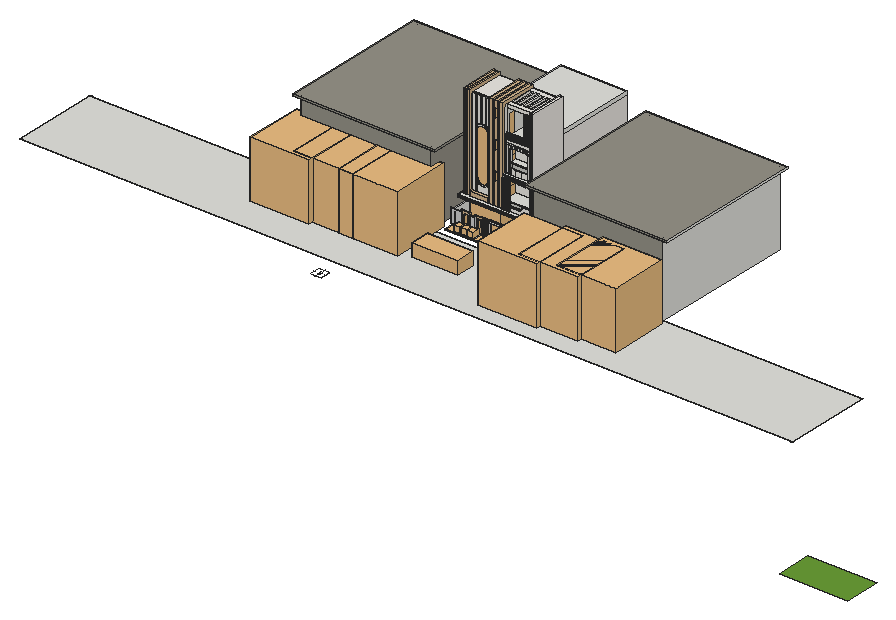
# SketchUp Ruby script. Lengths in inches.
U = 1.inch
M = Sketchup.active_model
def pt(a) = Geom::Point3d.new(a.map { |v| v * U })
def face(e, loops, mat)
  f = e.add_face(loops[0].map { |a| pt(a) })
  loops[1..].each { |l| e.add_face(l.map { |a| pt(a) }).erase! }
  f.material = f.back_material = mat if mat
  f
end
# faces: each face lists its corners as indices into pts; further lists are holes
def faces(e, pts, list, mat = nil) = list.each { |f| face(e, (f[0].is_a?(Array) ? f : [f]).map { |l| l.map { |i| pts[i] } }, mat) }
# xy, xz, yz: faces in a plane at the given z, y or x. An outline is a flat list of corners, or four numbers for a rectangle; further outlines are holes
def ring(l) = l.size == 4 ? [[l[0], l[1]], [l[2], l[1]], [l[2], l[3]], [l[0], l[3]]] : l.each_slice(2).to_a
def flat(e, list, mat, &to3) = list.each { |f| face(e, (f[0].is_a?(Array) ? f : [f]).map { |l| ring(l).map { |u, v| to3.(u, v) } }, mat) }
def xy(e, z, list, mat = nil) = flat(e, list, mat) { |x, y| [x, y, z] }
def xz(e, y, list, mat = nil) = flat(e, list, mat) { |x, z| [x, y, z] }
def yz(e, x, list, mat = nil) = flat(e, list, mat) { |y, z| [x, y, z] }
def lines(e, pts, list) = list.each { |a, b| e.add_line(pt(pts[a]), pt(pts[b])) }
# prism: a flat outline (further loops are holes) pulled along v
def prism(e, loops, v, mat = nil)
  f = face(e, loops, mat); d = Geom::Vector3d.new(v.map { |x| x * U })
  f.pushpull(f.normal.samedirection?(d) ? d.length : -d.length)
end
def box(e, o, s, mat = nil) = prism(e, [[o, [o[0] + s[0], o[1], o[2]], [o[0] + s[0], o[1] + s[1], o[2]], [o[0], o[1] + s[1], o[2]]]], [0, 0, s[2]], mat)
def at(x, y, z, deg = 0) = Geom::Transformation.translation(pt([x, y, z])) * Geom::Transformation.rotation(ORIGIN, Z_AXIS, deg.degrees)
def axes(o, x, y, z) = Geom::Transformation.new([*x, 0, *y, 0, *z, 0, *pt(o).to_a, 1])
def part(name) = M.definitions.add(name)
# library, detail: a bought-in or finely detailed component or shape, given as its bounding box
def library(name, o, s) = part(name).tap { |d| box(d.entities, o, s) }
def detail(e, o, s) = box(e.add_group.entities, o, s)
def put(e, d, t, mat = nil) = e.add_instance(d, t).tap { |i| i.material = mat if mat }
def group(e, t, mat = nil) = e.add_group.tap { |g| g.transformation = t; g.material = mat if mat }.entities
root = M.entities
M.materials.add("0025 AP L164 WHITE BUTTER").color = [234, 231, 225]
M.materials.add("Glass_Tinted_Gray").color = [0, 0, 0]
M.materials["Glass_Tinted_Gray"].alpha = 0.125
M.materials.add("[0035_Tan]").color = [210, 180, 140]
M.materials.add("[0133_Gray]").color = [128, 128, 128]
M.materials.add("[0135_DarkGray]").color = [81, 81, 81]
M.materials.add("[Carrera Marble]").color = [207, 207, 207]
M.materials.add("[Color_000]").color = [255, 255, 255]
M.materials.add("[Formica Graystone]").color = [149, 146, 135]
M.materials.add("[Grass Dark Green]").color = [106, 157, 55]
M.materials.add("[Mirror 02]").color = [229, 229, 229]
M.materials.add("[Terrazzo Light Blue]").color = [196, 214, 227]
M.materials.add("[Translucent_Glass_Gray]").color = [128, 128, 128]
M.materials["[Translucent_Glass_Gray]"].alpha = 0.5
M.materials.add("[Wood Cherry Original]").color = [152, 86, 42]
c1 = library("Auto cadd.dwg",[0,0,0],[290.55,512.6,0.01])
c2 = part("column")
box(c2.entities,[0,0,0],[12,12,120])
c3 = library("door58",[0,0,0],[34.0625,4.69,78.29])
c4 = part("PENTEK_RP Fineline 50S_Sliding_DoorCase_E1")
box(c4.entities,[0,0,0],[1.51,3.66,99.27],"[0135_DarkGray]")
c5 = part("PENTEK_RP Fineline 50S_SlidingDooe_Case_E2")
box(c5.entities,[0,0,0],[96.25,3.66,1.51],"[0135_DarkGray]")
c6 = part("pentek_RP Fineline 50S_SlidingDoor_Case")
put(c6.entities,c4,at(97.76,0,0))
put(c6.entities,c5,at(1.51,0,0))
put(c6.entities,c4,at(0,0,0))
put(c6.entities,c5,at(1.51,0,97.76))
c7 = part("PENTEK_RP Fineline 50S_SlidingDoor_GlazingBead_2")
box(c7.entities,[0,0,0],[0.56,0.59,94.39],"[0135_DarkGray]")
c8 = part("PENTEK_RP Fineline 50S_SlidingDoor_Glass")
box(c8.entities,[0,0,0],[46.58,0.16,94.39],"Glass_Tinted_Gray")
c9 = part("PENTEK_RP Fineline 50S_SlidingDoor_GlazingBead")
box(c9.entities,[0,0,0],[45.47,0.59,0.56],"[0135_DarkGray]")
c10 = part("PENTEK_RP Fineline 50S_SlidingDoor_Leaf_E1")
xy(c10.entities,0,[[0,0,0.93,1.97],[0.93,1.57,1.49,1.97]],"[0135_DarkGray]")
xy(c10.entities,96.25,[[0,0,0.93,0,0.93,1.57,1.49,1.57,1.49,1.97,0,1.97]],"[0135_DarkGray]")
xz(c10.entities,0,[[0,0,0.93,96.25]],"[0135_DarkGray]")
xz(c10.entities,1.57,[[0.93,0,1.49,95.32],[0.93,95.32,1.49,96.25]],"[0135_DarkGray]")
xz(c10.entities,1.97,[[0,0,1.49,96.25]],"[0135_DarkGray]")
yz(c10.entities,0,[[0,0,1.97,96.25]],"[0135_DarkGray]")
yz(c10.entities,0.93,[[0,0,1.57,0.93],[0,0.93,1.57,95.32],[0,95.32,1.57,96.25]],"[0135_DarkGray]")
yz(c10.entities,1.49,[[1.57,0,1.97,95.32],[1.57,95.32,1.97,96.25]],"[0135_DarkGray]")
c11 = part("PENTEK_RP Fineline 50S_SlidingDoor_Leaf_E2")
xy(c11.entities,0,[[0,0,0,1.57,0.56,1.57,0.56,1.97,46.02,1.97,46.02,1.57,46.58,1.57,46.58,0]],"[0135_DarkGray]")
xy(c11.entities,0.93,[[0,0,46.58,1.57]],"[0135_DarkGray]")
xy(c11.entities,1.49,[[0.56,1.57,46.02,1.97]],"[0135_DarkGray]")
xz(c11.entities,0,[[0,0,46.58,0.93]],"[0135_DarkGray]")
xz(c11.entities,1.57,[[0,0,0.56,0.93],[46.02,0,46.58,0.93],[0.56,0.93,46.02,1.49]],"[0135_DarkGray]")
xz(c11.entities,1.97,[[0.56,0,46.02,1.49]],"[0135_DarkGray]")
yz(c11.entities,0,[[0,0,1.57,0.93]],"[0135_DarkGray]")
yz(c11.entities,0.56,[[1.57,0,1.97,0.93],[1.57,0.93,1.97,1.49]],"[0135_DarkGray]")
yz(c11.entities,46.02,[[1.57,0,1.97,0.93],[1.57,0.93,1.97,1.49]],"[0135_DarkGray]")
yz(c11.entities,46.58,[[0,0,1.57,0.93]],"[0135_DarkGray]")
c12 = part("PENTEK_RP Fineline S_SlidingDoor_Leaf1")
put(c12.entities,c7,at(0.93,0,0.93))
put(c12.entities,c7,at(46.96,0,0.93))
put(c12.entities,c8,at(1.49,1.42,0.93))
put(c12.entities,c9,at(1.49,0,0.93))
put(c12.entities,c8,at(1.49,0.59,0.93),"[Terrazzo Light Blue]")
put(c12.entities,c10,at(0,0,0))
put(c12.entities,c10,axes([48.44,0,0],[-1,0,0],[0,1,0],[0,0,1]))
put(c12.entities,c11,axes([0.93,0,96.25],[1,0,0],[0,1,0],[0,0,-1]))
put(c12.entities,c11,at(0.93,0,0))
put(c12.entities,c9,at(1.49,0,94.77))
c13 = part("PENTEK_RP Fineline 50S_SlidingDoor_Leaf2")
put(c13.entities,c8,at(1.49,1.42,0.93))
put(c13.entities,c9,at(1.49,0,94.77))
put(c13.entities,c7,at(46.96,0,0.93))
put(c13.entities,c8,at(1.49,0.59,0.93),"[Mirror 02]")
put(c13.entities,c7,at(0.93,0,0.93))
put(c13.entities,c10,at(0,0,0))
put(c13.entities,c10,axes([48.44,0,0],[-1,0,0],[0,1,0],[0,0,1]))
put(c13.entities,c9,at(1.49,0,0.93))
put(c13.entities,c11,axes([0.93,0,96.25],[1,0,0],[0,1,0],[0,0,-1]))
put(c13.entities,c11,at(0.93,0,0))
c14 = part("PENTEK - Slimmest Steel Sliding Door / Window\#1")
put(c14.entities,c6,at(0,-1.88,-0.09))
put(c14.entities,c12,at(1.51,-2.27,1.42))
put(c14.entities,c13,at(49.32,-0.3,1.42))
c15 = part("window_2")
xy(c15.entities,0,[[-16,-4,16,0]],"[Color_000]")
xy(c15.entities,2,[[-14,-4,-5.25,0],[-4.25,-4,4.25,0],[5.25,-4,14,0]],"[Color_000]")
xy(c15.entities,10.75,[[-14,-4,-5.25,0],[-4.25,-4,4.25,0],[5.25,-4,14,0]],"[Color_000]")
xy(c15.entities,11.75,[[-14,-4,-5.25,0],[-4.25,-4,4.25,0],[5.25,-4,14,0]],"[Color_000]")
xy(c15.entities,20,[[-14,-4,-5.25,0],[-4.25,-4,4.25,0],[5.25,-4,14,0]],"[Color_000]")
xy(c15.entities,21,[[-14,-4,-5.25,0],[-4.25,-4,4.25,0],[5.25,-4,14,0]],"[Color_000]")
xy(c15.entities,29.25,[[-14,-4,-5.25,0],[-4.25,-4,4.25,0],[5.25,-4,14,0]],"[Color_000]")
xy(c15.entities,30.25,[[-14,-4,-5.25,0],[-4.25,-4,4.25,0],[5.25,-4,14,0]],"[Color_000]")
xy(c15.entities,39,[[-14,-4,-5.25,0],[-4.25,-4,4.25,0],[5.25,-4,14,0]],"[Color_000]")
xy(c15.entities,41,[[-16,-4,16,0]],"[Color_000]")
xz(c15.entities,-4,[[[-16,0,16,41],[-14,30.25,-5.25,39],[5.25,30.25,14,39],[5.25,2,14,10.75],[-14,2,-5.25,10.75],[-4.25,30.25,4.25,39],[-4.25,2,4.25,10.75],[5.25,21,14,29.25],[5.25,11.75,14,20],[-14,21,-5.25,29.25],[-14,11.75,-5.25,20],[-4.25,21,4.25,29.25],[-4.25,11.75,4.25,20]]],"[Color_000]")
xz(c15.entities,0,[[[-16,0,16,41],[5.25,30.25,14,39],[-14,30.25,-5.25,39],[5.25,2,14,10.75],[-14,2,-5.25,10.75],[-4.25,30.25,4.25,39],[-4.25,2,4.25,10.75],[5.25,21,14,29.25],[5.25,11.75,14,20],[-14,21,-5.25,29.25],[-14,11.75,-5.25,20],[-4.25,21,4.25,29.25],[-4.25,11.75,4.25,20]]],"[Color_000]")
xz(c15.entities,0,[[-14,2,-5.25,10.75],[-4.25,2,4.25,10.75],[5.25,2,14,10.75],[-14,11.75,-5.25,20],[-4.25,11.75,4.25,20],
  [5.25,11.75,14,20],[-14,21,-5.25,29.25],[-4.25,21,4.25,29.25],[5.25,21,14,29.25],[-14,30.25,-5.25,39],
  [-4.25,30.25,4.25,39],[5.25,30.25,14,39]],"[Translucent_Glass_Gray]")
yz(c15.entities,-16,[[-4,0,0,41]],"[Color_000]")
yz(c15.entities,-14,[[-4,2,0,10.75],[-4,11.75,0,20],[-4,21,0,29.25],[-4,30.25,0,39]],"[Color_000]")
yz(c15.entities,-5.25,[[-4,2,0,10.75],[-4,11.75,0,20],[-4,21,0,29.25],[-4,30.25,0,39]],"[Color_000]")
yz(c15.entities,-4.25,[[-4,2,0,10.75],[-4,11.75,0,20],[-4,21,0,29.25],[-4,30.25,0,39]],"[Color_000]")
yz(c15.entities,4.25,[[-4,2,0,10.75],[-4,11.75,0,20],[-4,21,0,29.25],[-4,30.25,0,39]],"[Color_000]")
yz(c15.entities,5.25,[[-4,2,0,10.75],[-4,11.75,0,20],[-4,21,0,29.25],[-4,30.25,0,39]],"[Color_000]")
yz(c15.entities,14,[[-4,2,0,10.75],[-4,11.75,0,20],[-4,21,0,29.25],[-4,30.25,0,39]],"[Color_000]")
yz(c15.entities,16,[[-4,0,0,41]],"[Color_000]")
c16 = part("Square post")
xy(c16.entities,0,[[0,-3,3,0]])
xy(c16.entities,120,[[0,-3,3,0]],"[0133_Gray]")
xz(c16.entities,-3,[[0,0,3,120]],"[0133_Gray]")
xz(c16.entities,0,[[0,0,3,120]],"[0133_Gray]")
yz(c16.entities,0,[[-3,0,0,120]])
yz(c16.entities,3,[[-3,0,0,120]],"[0133_Gray]")
c17 = library("3d+gate",[66.37,49.16,0.6875],[138,1.5,69])
c18 = library("Quince Tree 003",[-75.25,-60.68,-2.4],[147.3,122.84,127.75])
c19 = library("Bottlebrush Tree 15-12",[-86.81,-76.76,-0.05],[168.11,159.05,130.9])
c20 = library("Dome Light",[-12,-12,0],[24,24,12])
c21 = library("Cigar Tree 54-39",[-131.92,-127.4375,0],[258.61,255.15,252.0625])
c22 = part("Group276\#1")
p = [[24,24,0],[24,0,0],[-24,-24,0],[-24,0,0],[-24,24,0],[0,24,0],
  [24,-24,0],[0,-24,0],[5.4,5.4,0],[5.22,6.8,0],[3.82,9.22,0],[2.7,10.08,0],
  [3.82,-9.22,0],[4.68,-8.1,0],[-1.4,-0.18,0],[-2.7,-0.72,0],[4.68,-2.7,0],[3.82,-1.58,0],
  [-4.68,-2.7,0],[-5.22,-4,0],[0,-19.2,0],[1.4,10.62,0],[-5.4,5.4,0],[-5.22,4,0],
  [-3.82,9.22,0],[-4.68,8.1,0],[4.68,8.1,0],[-2.7,-10.08,0],[-1.4,-10.62,0],[5.22,-4,0],
  [-2.7,10.08,0],[-5.4,-5.4,0],[-5.22,-6.8,0],[0,-10.8,0],[0,10.8,0],[-1.4,10.62,0],
  [5.22,4,0],[3.82,1.58,0],[4.68,2.7,0],[-4.68,-8.1,0],[1.4,-10.62,0],[2.7,-10.08,0],
  [0,28.8,0],[19.2,0,0],[5.22,-6.8,0],[0,0,0],[-3.82,-1.58,0],[0,-3.6,0],
  [-5.22,6.8,0],[5.4,-5.4,0],[2.7,0.72,0],[-4.68,2.7,0],[-3.82,1.58,0],[-3.82,-9.22,0],
  [0,3.6,0],[1.4,0.18,0],[-28.8,0,0],[0,-28.8,0],[0,19.2,0],[28.8,0,0],
  [-19.2,0,0]]
lines(c22.entities,p,[[0,1],[2,3],[4,5],[6,7],[8,9],[10,11],[12,13],[14,15],[16,17],[18,19],[20,7],[11,21],
  [22,23],[24,25],[26,10],[27,28],[29,16],[30,24],[19,31],[31,32],[28,33],[34,35],[36,8],[9,26],
  [37,38],[35,30],[32,39],[21,34],[40,41],[42,5],[43,1],[13,44],[45,14],[46,18],[45,47],[25,48],
  [49,29],[50,37],[48,22],[51,52],[33,40],[39,53],[45,54],[41,12],[44,49],[38,36],[55,45],[55,50],
  [53,27],[15,46],[23,51],[56,3],[1,6],[3,4],[5,0],[7,2],[7,57],[5,58],[1,59],[3,60]])
c23 = part("Infinite Plane")
put(c23.entities,c22,at(0,0,0))
c24 = library("Car 033",[-43.24,-98.19,-1.29],[86.48,201.64,57.79])
c25 = library("Group\#6",[0,0,0],[78,136.23,163.57])
c26 = part("Group\#7")
xy(c26.entities,0,[[0,0,0,420.68,290.55,420.68,290.55,0,278.55,0,278.55,9,281.55,9,281.55,411.68,9,411.68,9,9,242.55,9,242.55,0]])
xy(c26.entities,36,[[146.55,0,182.55,9],[194.55,0,230.55,9]])
xy(c26.entities,84,[[146.55,0,182.55,9],[194.55,0,230.55,9],[242.55,0,278.55,9]])
xy(c26.entities,120,[[[0,0,290.55,420.68],[9,9,281.55,411.68]]])
xz(c26.entities,0,[[[0,0,242.55,0,242.55,84,278.55,84,278.55,0,290.55,0,290.55,120,0,120],[194.55,36,230.55,84],[146.55,36,182.55,84]]])
xz(c26.entities,9,[[[9,0,9,120,281.55,120,281.55,0,278.55,0,278.55,84,242.55,84,242.55,0],[194.55,36,230.55,84],[146.55,36,182.55,84]]])
xz(c26.entities,411.68,[[9,0,281.55,120]])
xz(c26.entities,420.68,[[0,0,290.55,120]])
yz(c26.entities,0,[[0,0,420.68,120]])
yz(c26.entities,9,[[9,0,411.68,120]])
yz(c26.entities,146.55,[[0,36,9,84]])
yz(c26.entities,182.55,[[0,36,9,84]])
yz(c26.entities,194.55,[[0,36,9,84]])
yz(c26.entities,230.55,[[0,36,9,84]])
yz(c26.entities,242.55,[[0,0,9,84]])
yz(c26.entities,278.55,[[0,0,9,84]])
yz(c26.entities,281.55,[[9,0,411.68,120]])
yz(c26.entities,290.55,[[0,0,420.68,120]])
c27 = part("Group\#13")
prism(c27.entities,[[[12,0,0],[12,0,402],[12,154,402],[12,154,414],[12,-12,414],[12,-12,0]]],[-12,0,0])
c28 = library("Group\#27",[0,-1,0],[52,1,231.95])
c29 = part("Group\#30")
box(c29.entities,[-24,-4,0],[42,4,66])
c30 = library("Group\#35",[0,-48,0],[362.55,48,4])
c31 = library("Group\#79",[0,0,0],[8.93,9.09,32.75])
c32 = library("Group\#80",[0,0.1875,0],[8.9,8.9,12.8125])
c33 = library("Group\#82",[0,0,-2],[12,12,2])
xy(root,0,[[3937.03,0,4237.78,156.4375]],"[Grass Dark Green]")
put(root,c1,at(1572.76,1240.67,0))
put(root,c2,at(1615.1,1716.58,4))
put(root,c2,at(1711.1,1716.58,4))
put(root,c2,at(1807.1,1716.58,4))
put(root,c2,at(1615.1,1620.58,4))
put(root,c2,at(1711.1,1620.58,4))
put(root,c2,at(1807.1,1620.58,4))
put(root,c2,at(1615.1,1524.58,4))
put(root,c2,at(1807.1,1524.58,4))
put(root,c2,at(1711.1,1524.58,4))
put(root,c2,at(1711.1,1428.58,4))
put(root,c2,at(1807.1,1428.58,4))
put(root,c2,at(1615.1,1428.58,4))
put(root,c2,at(1807.1,1332.58,4))
put(root,c2,at(1711.1,1332.58,4))
put(root,c2,at(1615.1,1332.58,4))
put(root,c3,axes([1815.31,1332.58,134],[1.05686,0,0],[0,1,0],[0,0,1.07289]))
put(root,c3,axes([1815.31,1332.58,268],[1.05686,0,0],[0,1,0],[0,0,1.07289]))
put(root,c3,axes([1740.76,1257.2,402],[0,1.05686,0],[-1,0,0],[0,0,1.07289]))
put(root,c14,axes([1767.31,1333.85,304.04],[0.36264,0,0],[0,0.73,0],[0,0,0.48352]))
put(root,c14,axes([1767.31,1333.85,170.04],[0.36264,0,0],[0,0.73,0],[0,0,0.48352]))
put(root,c15,axes([1737.31,1336.58,170],[1.125,0,0],[0,1,0],[0,0,1.17073]))
put(root,c15,axes([1737.31,1336.58,304],[1.125,0,0],[0,1,0],[0,0,1.17073]))
put(root,c16,at(1745.76,1218.67,134))
put(root,c16,at(1751.76,1218.67,134))
put(root,c16,at(1757.76,1218.67,134))
put(root,c16,at(1763.76,1218.67,134))
put(root,c16,at(1769.76,1218.67,134))
put(root,c16,at(1775.76,1218.67,134))
put(root,c17,axes([1634.89,1160.37,3.4],[1,0,0],[0,1,0],[0,0,0.86957]))
put(root,c18,axes([1884.24,1178.29,10.6],[0.25089,0,0],[0,0.25089,0],[0,0,0.25089]))
put(root,c19,axes([1586.8,1180.32,7.26],[0.18,0,0],[0,0.18,0],[0,0,0.18]))
put(root,c19,axes([1614.92,1180.32,7.26],[0.18,0,0],[0,0.18,0],[0,0,0.18]))
put(root,c19,axes([1643.05,1180.32,7.26],[0.18,0,0],[0,0.18,0],[0,0,0.18]))
put(root,c20,at(2213.9375,956.5,0.1))
put(root,c21,at(2083.7,949.61,0.1))
put(root,c21,at(1394.86,1047.6,0.1))
put(root,c21,at(1196.34,1048.32,0.1))
put(root,c21,at(1019.91,1029.81,0.1))
put(root,c21,at(2251.58,967.31,0.1))
put(root,c21,at(2402.93,986.31,0.1))
put(root,c23,at(1379.73,670.47,-8.625),"[Grass Dark Green]")
put(root,c24,at(1668.94,986.24,0.1,90))
g1 = group(root,at(1572.76,1240.67,0))
box(g1,[-36,-29.61,0],[362.55,578.21,4])
g2 = group(root,at(1572.76,1240.67,120))
xy(g2,0,[[-12,-36,-12,9.78,136.23,9.78,136.23,91.92,0,91.92,0,9.78,-12,9.78,-12,512.6,326.55,512.6,326.55,-36]])
xy(g2,3,[[-12,-36,326.55,-34],[-12,-34,-10,512.6],[324.55,-34,326.55,512.6]])
xy(g2,11,[[-12,-36,326.55,-34],[-12,-34,-10,512.6],[324.55,-34,326.55,512.6]])
xy(g2,14,[[[-12,-36,326.55,512.6],[0,9.78,136.23,91.92]]])
xz(g2,-36,[[-12,0,326.55,3],[-12,11,326.55,14]])
xz(g2,-34,[[-10,3,324.55,11]])
xz(g2,9.78,[[0,0,136.23,14]])
xz(g2,91.92,[[0,0,136.23,14]])
xz(g2,512.6,[[-12,0,-12,3,-10,3,-10,11,-12,11,-12,14,326.55,14,326.55,11,324.55,11,324.55,3,326.55,3,326.55,0]])
yz(g2,-12,[[-36,0,512.6,3],[-36,11,512.6,14]])
yz(g2,-10,[[-34,3,512.6,11]])
yz(g2,0,[[9.78,0,91.92,14]])
yz(g2,136.23,[[9.78,0,91.92,14]])
yz(g2,324.55,[[-34,3,512.6,11]])
yz(g2,326.55,[[-36,0,512.6,3],[-36,11,512.6,14]])
put(root,c25,at(1708.99,1254.58,4,90))
put(root,c26,at(1572.76,1332.58,134),"0025 AP L164 WHITE BUTTER")
g3 = group(root,at(1572.76,1240.67,254))
xy(g3,0,[[173,-22,173,0,0,0,0,9.78,136.23,9.78,136.23,91.92,0,91.92,0,512.6,290.55,512.6,290.55,-22]],"[Wood Cherry Original]")
xy(g3,3,[[173,-22,290.55,-19]])
xy(g3,11,[[173,-22,290.55,-19]])
xy(g3,14,[[173,-22,290.55,-22,290.55,512.6,0,512.6,0,91.92,136.23,91.92,136.23,9.78,0,9.78,0,0,173,0]])
xz(g3,-22,[[173,0,290.55,3],[173,11,290.55,14]])
xz(g3,-19,[[173,3,290.55,11]])
xz(g3,0,[[0,0,173,14]])
xz(g3,9.78,[[0,0,136.23,14]])
xz(g3,91.92,[[0,0,136.23,14]])
xz(g3,512.6,[[0,0,290.55,14]])
yz(g3,0,[[0,0,9.78,14],[9.78,0,91.92,14],[91.92,0,512.6,14]])
yz(g3,136.23,[[9.78,0,91.92,14]])
yz(g3,173,[[-22,0,-22,3,-19,3,-19,11,-22,11,-22,14,0,14,0,0]])
yz(g3,290.55,[[-22,0,512.6,0,512.6,14,-22,14,-22,11,-19,11,-19,3,-22,3]])
g4 = group(root,at(1572.76,1240.67,388))
xy(g4,0,[[173,-6,173,0,0,0,0,9.78,136.23,9.78,136.23,91.92,0,91.92,0,512.6,290.55,512.6,290.55,-6]],"[Wood Cherry Original]")
xy(g4,14,[[173,-6,290.55,-6,290.55,512.6,0,512.6,0,91.92,136.23,91.92,136.23,9.78,0,9.78,0,0,173,0]])
xz(g4,-6,[[173,0,290.55,14]],"0025 AP L164 WHITE BUTTER")
xz(g4,0,[[0,0,173,14]])
xz(g4,9.78,[[0,0,136.23,14]])
xz(g4,91.92,[[0,0,136.23,14]])
xz(g4,512.6,[[0,0,290.55,14]])
yz(g4,0,[[0,0,9.78,14],[9.78,0,91.92,14],[91.92,0,512.6,14]])
yz(g4,136.23,[[9.78,0,91.92,14]])
yz(g4,173,[[-6,0,0,14]])
yz(g4,290.55,[[-6,0,512.6,14]])
put(root,c26,at(1572.76,1332.58,268),"0025 AP L164 WHITE BUTTER")
put(root,c25,at(1708.99,1254.58,124,90))
put(root,c25,at(1708.99,1254.58,244,90))
g5 = group(root,at(1572.76,1240.67,402))
xy(g5,0,[[0,0,0,144,168,144,168,52.54,159,52.54,159,135,9,135,9,9,159,9,159,16.54,168,16.54,168,0]])
xy(g5,84,[[159,16.54,168,52.54]])
xy(g5,120,[[[0,0,168,144],[9,9,159,135]]])
xz(g5,0,[[0,0,168,120]])
xz(g5,9,[[9,0,159,120]])
xz(g5,16.54,[[159,0,168,84]])
xz(g5,52.54,[[159,0,168,84]])
xz(g5,135,[[9,0,159,120]])
xz(g5,144,[[0,0,168,120]])
yz(g5,0,[[0,0,144,120]])
yz(g5,9,[[9,0,135,120]])
yz(g5,159,[[9,0,9,120,135,120,135,0,52.54,0,52.54,84,16.54,84,16.54,0]])
yz(g5,168,[[0,0,16.54,0,16.54,84,52.54,84,52.54,0,144,0,144,120,0,120]])
g6 = group(root,at(1863.31,1240.67,134))
xy(g6,0,[[0,-22,0,144,14,144,14,-22,9,-22,9,-20,5,-20,5,-22]])
xy(g6,414,[[0,-22,5,-22,5,-20,9,-20,9,-22,14,-22,14,144,0,144]],"0025 AP L164 WHITE BUTTER")
xz(g6,-22,[[0,0,5,414],[9,0,14,414]],"0025 AP L164 WHITE BUTTER")
xz(g6,-20,[[5,0,9,414]],"[0133_Gray]")
xz(g6,144,[[0,0,14,414]])
yz(g6,0,[[-22,0,144,414]],"0025 AP L164 WHITE BUTTER")
yz(g6,5,[[-22,0,-20,414]],"[0133_Gray]")
yz(g6,9,[[-22,0,-20,414]],"[0133_Gray]")
yz(g6,14,[[-22,0,144,414]],"0025 AP L164 WHITE BUTTER")
g7 = group(root,at(1572.76,1240.67,522),"0025 AP L164 WHITE BUTTER")
prism(g7,[[[0,144,0],[290.55,144,0],[290.55,0,0],[0,0,0]],[[180,24,0],[192,24,0],[192,120,0],[180,120,0]],[[204,24,0],[216,24,0],[216,120,0],[204,120,0]],[[228,24,0],[240,24,0],[240,120,0],[228,120,0]],[[252,24,0],[264,24,0],[264,120,0],[252,120,0]],[[276,24,0],[288,24,0],[288,120,0],[276,120,0]]],[0,0,14])
g8 = group(root,at(1572.76,1240.67,134),"0025 AP L164 WHITE BUTTER")
xy(g8,0,[[0,-10,0,0,173,0,173,-10,132,-10,132,-8,129,-8,129,-10,111,-10,111,-8,108,-8,108,-10,48,-10,48,-8,45,-8,45,-10,27,-10,27,-8,24,-8,24,-10]])
xy(g8,402,[[0,-10,24,-10,24,-8,27,-8,27,-10,45,-10,45,-8,48,-8,48,-10,66,-10,66,-8,69,-8,69,-10,87,-10,87,-8,90,-8,90,-10,108,-10,108,-8,111,-8,111,-10,129,-10,129,-8,132,-8,132,-10,173,-10,173,0,0,0]])
xz(g8,-16,[[[78,52,84.86,52.77,91.37,55.06,97.21,58.74,102.08,63.63,105.74,69.48,108,76,108,268,105.74,274.52,102.08,280.37,97.21,285.26,91.37,288.94,90,289.42,87,290.47,84.86,291.23,78,292,71.14,291.23,69,290.47,66,289.42,64.63,288.94,58.79,285.26,53.92,280.37,50.26,274.52,48,268,48,76,50.26,69.48,53.92,63.63,58.79,58.74,64.63,55.06,71.14,52.77],[78,56.03,72.04,56.7,66.38,58.68,61.31,61.88,57.07,66.13,53.89,71.22,52,76.67,52,267.33,53.89,272.78,57.07,277.87,61.31,282.12,66.38,285.32,72.04,287.3,78,287.97,83.96,287.3,89.62,285.32,94.69,282.12,98.93,277.87,102.11,272.78,104,267.33,104,76.67,102.11,71.22,98.93,66.13,94.69,61.88,89.62,58.68,83.96,56.7]]])
xz(g8,-10,[[0,0,24,402],[27,0,45,402],[48,0,108,0,108,76,105.74,69.48,102.08,63.63,97.21,58.74,91.37,55.06,84.86,52.77,78,52,71.14,52.77,64.63,55.06,58.79,58.74,53.92,63.63,50.26,69.48,48,76],[111,0,129,402],[132,0,173,402],
  [48,268,50.26,274.52,53.92,280.37,58.79,285.26,64.63,288.94,66,289.42,66,402,48,402],[108,268,108,402,90,402,90,289.42,91.37,288.94,97.21,285.26,102.08,280.37,105.74,274.52],[69,290.47,71.14,291.23,78,292,84.86,291.23,87,290.47,87,402,69,402]])
xz(g8,-8,[[24,0,27,402]])
xz(g8,-8,[[45,0,48,402],[108,0,111,402],[129,0,132,402],[66,289.42,69,290.47,69,402,66,402],[90,289.42,90,402,87,402,87,290.47]],"[0133_Gray]")
xz(g8,0,[[[0,0,173,402],[78,56.03,83.96,56.7,89.62,58.68,94.69,61.88,98.93,66.13,102.11,71.22,104,76.67,104,267.33,102.11,272.78,98.93,277.87,94.69,282.12,89.62,285.32,83.96,287.3,78,287.97,72.04,287.3,66.38,285.32,61.31,282.12,57.07,277.87,53.89,272.78,52,267.33,52,76.67,53.89,71.22,57.07,66.13,61.31,61.88,66.38,58.68,72.04,56.7]]])
yz(g8,0,[[-10,0,0,402]])
yz(g8,24,[[-10,0,-8,402]])
yz(g8,27,[[-10,0,-8,402]])
yz(g8,45,[[-10,0,-8,402]],"[0133_Gray]")
yz(g8,48,[[-10,0,-8,76],[-16,76,-8,268]])
yz(g8,48,[[-10,268,-8,402]],"[0133_Gray]")
yz(g8,52,[[-16,76.67,0,267.33]])
yz(g8,66,[[-10,289.42,-8,402]],"[0133_Gray]")
yz(g8,69,[[-10,290.47,-8,402]],"[0133_Gray]")
yz(g8,87,[[-10,290.47,-8,402]],"[0133_Gray]")
yz(g8,90,[[-10,289.42,-8,402]],"[0133_Gray]")
yz(g8,104,[[-16,76.67,0,267.33]])
yz(g8,108,[[-10,0,-8,76],[-16,76,-8,268]])
yz(g8,108,[[-10,268,-8,402]],"[0133_Gray]")
yz(g8,111,[[-10,0,-8,402]],"[0133_Gray]")
yz(g8,129,[[-10,0,-8,402]],"[0133_Gray]")
yz(g8,132,[[-10,0,-8,402]],"[0133_Gray]")
yz(g8,173,[[-10,0,0,402]])
p = [[71.14,-10,52.77],[78,-10,52],[78,-16,52],[71.14,-16,52.77],[84.86,-10,52.77],[84.86,-16,52.77],
  [64.63,-10,55.06],[64.63,-16,55.06],[91.37,-10,55.06],[91.37,-16,55.06],[58.79,-10,58.74],[58.79,-16,58.74],
  [97.21,-10,58.74],[97.21,-16,58.74],[72.04,0,56.7],[72.04,-16,56.7],[78,-16,56.03],[78,0,56.03],
  [83.96,-16,56.7],[83.96,0,56.7],[66.38,0,58.68],[66.38,-16,58.68],[89.62,-16,58.68],[89.62,0,58.68],
  [53.92,-10,63.63],[53.92,-16,63.63],[61.31,0,61.88],[61.31,-16,61.88],[94.69,-16,61.88],[94.69,0,61.88],
  [102.08,-10,63.63],[102.08,-16,63.63],[57.07,0,66.13],[57.07,-16,66.13],[98.93,-16,66.13],[98.93,0,66.13],
  [50.26,-10,69.48],[50.26,-16,69.48],[105.74,-10,69.48],[105.74,-16,69.48],[53.89,0,71.22],[53.89,-16,71.22],
  [102.11,-16,71.22],[102.11,0,71.22],[48,-10,76],[48,-16,76],[108,-10,76],[108,-16,76],
  [52,0,76.67],[52,-16,76.67],[104,-16,76.67],[104,0,76.67],[53.89,0,272.78],[53.89,-16,272.78],
  [52,-16,267.33],[52,0,267.33],[104,0,267.33],[104,-16,267.33],[102.11,-16,272.78],[102.11,0,272.78],
  [50.26,-10,274.52],[48,-10,268],[48,-16,268],[50.26,-16,274.52],[108,-10,268],[105.74,-10,274.52],
  [105.74,-16,274.52],[108,-16,268],[57.07,0,277.87],[57.07,-16,277.87],[98.93,-16,277.87],[98.93,0,277.87],
  [53.92,-10,280.37],[53.92,-16,280.37],[102.08,-10,280.37],[102.08,-16,280.37],[61.31,0,282.12],[61.31,-16,282.12],
  [94.69,-16,282.12],[94.69,0,282.12],[58.79,-10,285.26],[58.79,-16,285.26],[97.21,-10,285.26],[97.21,-16,285.26],
  [66.38,0,285.32],[66.38,-16,285.32],[89.62,-16,285.32],[89.62,0,285.32],[64.63,-10,288.94],[64.63,-16,288.94],
  [72.04,0,287.3],[72.04,-16,287.3],[83.96,-16,287.3],[83.96,0,287.3],[91.37,-10,288.94],[91.37,-16,288.94],
  [78,0,287.97],[78,-16,287.97],[66,-10,289.42],[66,-16,289.42],[90,-10,289.42],[90,-16,289.42],
  [66,-8,289.42],[69,-16,290.47],[69,-10,290.47],[69,-8,290.47],[87,-8,290.47],[87,-10,290.47],
  [87,-16,290.47],[90,-8,289.42],[71.14,-10,291.23],[71.14,-16,291.23],[84.86,-10,291.23],[84.86,-16,291.23],
  [78,-10,292],[78,-16,292],[66,-10,288.94],[90,-10,288.94]]
faces(g8,p,[[0,1,2,3],[1,4,5,2],[6,0,3,7],[4,8,9,5],[10,6,7,11],[8,12,13,9],[14,15,16,17],[17,16,18,19],
  [20,21,15,14],[19,18,22,23],[24,10,11,25],[26,27,21,20],[23,22,28,29],[12,30,31,13],[32,33,27,26],[29,28,34,35],
  [36,24,25,37],[30,38,39,31],[40,41,33,32],[35,34,42,43],[44,36,37,45],[38,46,47,39],[48,49,41,40],[43,42,50,51],
  [52,53,54,55],[56,57,58,59],[60,61,62,63],[64,65,66,67],[68,69,53,52],[59,58,70,71],[72,60,63,73],[65,74,75,66],
  [76,77,69,68],[71,70,78,79],[80,72,73,81],[74,82,83,75],[84,85,77,76],[79,78,86,87],[88,80,81,89],[90,91,85,84],
  [87,86,92,93],[82,94,95,83],[96,97,91,90],[93,92,97,96],[98,88,89,99],[94,100,101,95],[102,98,99,103,104,105],[106,107,108,101,100,109],
  [110,104,103,111],[107,112,113,108],[114,110,111,115],[112,114,115,113]])
lines(g8,p,[[98,116],[100,117]])
put(root,c27,at(1572.76,1230.67,134),"[0035_Tan]")
put(root,c27,at(1587.76,1230.67,134),"[0035_Tan]")
g9 = group(root,at(1683.76,1230.67,134),"[0035_Tan]")
prism(g9,[[[0,0,402],[0,0,0],[0,-12,0],[0,-12,414],[0,154,414],[0,154,402]]],[18,0,0])
g10 = group(root,at(1705.76,1230.67,134),"[0035_Tan]")
prism(g10,[[[0,0,402],[0,0,0],[0,-12,0],[0,-12,414],[0,154,414],[0,154,402]]],[18,0,0])
p = [[0,0,402],[-1,0,402]]
lines(g10,p,[[0,1]])
g11 = group(root,at(1727.76,1230.67,134),"[0035_Tan]")
prism(g11,[[[0,0,402],[0,0,0],[0,-12,0],[0,-12,414],[0,154,414],[0,154,402]]],[18,0,0])
g12 = group(root,at(1745.76,1218.67,134))
g13 = group(g12,at(0,-2,0),"0025 AP L164 WHITE BUTTER")
xy(g13,0,[[0,2,117.55,6.5]])
xy(g13,18,[[0,2,75.55,5]])
xy(g13,36,[[87.55,2,117.55,6.5],[0,5,87.55,6.5]])
xz(g13,2,[[0,0,117.55,0,117.55,33,89.16,33,77.16,15,0,15],[0,15,77.16,15,89.16,33,117.55,33,117.55,36,87.55,36,75.55,18,0,18]])
xz(g13,5,[[0,34,86.22,34,87.55,36,0,36]])
xz(g13,5,[[0,18,75.55,18,86.22,34,0,34]],"Glass_Tinted_Gray")
xz(g13,6.5,[[0,0,117.55,36]],"Glass_Tinted_Gray")
yz(g13,0,[[2,0,2,18,5,18,5,36,6.5,36,6.5,0]])
yz(g13,117.55,[[2,0,6.5,36]])
p = [[86.22,5,34],[75.55,5,18],[75.55,2,18],[87.55,2,36],[87.55,5,36]]
faces(g13,p,[[0,1,2,3,4]])
g14 = group(root,at(1601.82,1230.67,134),"[0035_Tan]")
box(g14,[0,-12,0],[78.9375,12,20.3125])
g15 = group(root,at(1745.76,1240.67,268),"0025 AP L164 WHITE BUTTER")
xy(g15,0,[[0,-8,4.32,0],[113.23,-8,117.55,0],[4.32,-6,21.62,0],[21.62,-6,95.93,0],[95.93,-6,113.23,0]])
xy(g15,2,[[6.32,-6,19.62,-4],[97.93,-6,111.23,-4]])
xy(g15,105,[[30.27,-6,87.28,0]])
xy(g15,107,[[30.22,-6,87.33,-4]])
xy(g15,115,[[6.32,-6,111.23,-4]])
xy(g15,117,[[4.32,-8,113.23,-6]])
xy(g15,120,[[0,-8,117.55,0]])
xz(g15,-8,[[0,0,4.32,0,4.32,117,113.23,117,113.23,0,117.55,0,117.55,120,0,120]])
xz(g15,-6,[[[4.32,0,21.62,0,21.62,99,21.7,99.78,21.92,100.55,22.28,101.3,22.78,102,23.41,102.65,24.15,103.24,25.01,103.76,25.95,104.2,26.96,104.54,28.03,104.8,29.14,104.95,30.27,105,87.28,105,88.41,104.95,89.52,104.8,90.59,104.54,91.61,104.2,92.55,103.76,93.4,103.24,94.14,102.65,94.77,102,95.27,101.3,95.63,100.55,95.86,99.78,95.93,99,95.93,0,113.23,0,113.23,117,4.32,117],[6.32,2,6.32,115,111.23,115,111.23,2,97.93,2,97.93,99.09,97.83,100.16,97.51,101.27,97,102.32,96.31,103.28,95.49,104.14,94.54,104.89,93.49,105.53,92.35,106.05,91.14,106.47,89.89,106.76,88.59,106.94,87.33,107,30.22,107,28.96,106.94,27.67,106.76,26.41,106.47,25.2,106.05,24.0625,105.53,23.01,104.89,22.0625,104.14,21.24,103.28,20.56,102.32,20.04,101.27,19.72,100.16,19.62,99.09,19.62,2]]])
xz(g15,-4,[[6.32,2,19.62,2,19.62,99.09,19.72,100.16,20.04,101.27,20.56,102.32,21.24,103.28,22.0625,104.14,23.01,104.89,24.0625,105.53,25.2,106.05,26.41,106.47,27.67,106.76,28.96,106.94,30.22,107,87.33,107,88.59,106.94,89.89,106.76,91.14,106.47,92.35,106.05,93.49,105.53,94.54,104.89,95.49,104.14,96.31,103.28,97,102.32,97.51,101.27,97.83,100.16,97.93,99.09,97.93,2,111.23,2,111.23,115,6.32,115]])
xz(g15,0,[[[4.32,0,4.32,117,113.23,117,113.23,0,95.93,0,95.93,99,95.86,99.78,95.63,100.55,95.27,101.3,94.77,102,94.14,102.65,93.4,103.24,92.55,103.76,91.61,104.2,90.59,104.54,89.52,104.8,88.41,104.95,87.28,105,30.27,105,29.14,104.95,28.03,104.8,26.96,104.54,25.95,104.2,25.01,103.76,24.15,103.24,23.41,102.65,22.78,102,22.28,101.3,21.92,100.55,21.7,99.78,21.62,99,21.62,0],[6.32,2,19.62,2,19.62,99.09,19.72,100.16,20.04,101.27,20.56,102.32,21.24,103.28,22.0625,104.14,23.01,104.89,24.0625,105.53,25.2,106.05,26.41,106.47,27.67,106.76,28.96,106.94,30.22,107,87.33,107,88.59,106.94,89.89,106.76,91.14,106.47,92.35,106.05,93.49,105.53,94.54,104.89,95.49,104.14,96.31,103.28,97,102.32,97.51,101.27,97.83,100.16,97.93,99.09,97.93,2,111.23,2,111.23,115,6.32,115]]])
yz(g15,0,[[-8,0,0,120]])
yz(g15,4.32,[[-8,0,-6,117]])
yz(g15,6.32,[[-6,2,-4,115]])
yz(g15,19.62,[[-6,2,-4,99.09]])
yz(g15,21.62,[[-6,0,0,99]])
yz(g15,95.93,[[-6,0,0,99]])
yz(g15,97.93,[[-6,2,-4,99.09]])
yz(g15,111.23,[[-6,2,-4,115]])
yz(g15,113.23,[[-8,0,-6,117]])
yz(g15,117.55,[[-8,0,0,120]])
p = [[21.62,0,99],[21.7,0,99.78],[21.7,-6,99.78],[21.62,-6,99],[95.86,0,99.78],[95.93,0,99],
  [95.93,-6,99],[95.86,-6,99.78],[19.62,-6,99.09],[19.72,-6,100.16],[19.72,-4,100.16],[19.62,-4,99.09],
  [97.83,-6,100.16],[97.93,-6,99.09],[97.93,-4,99.09],[97.83,-4,100.16],[21.92,0,100.55],[21.92,-6,100.55],
  [95.63,0,100.55],[95.63,-6,100.55],[20.04,-6,101.27],[20.04,-4,101.27],[97.51,-6,101.27],[97.51,-4,101.27],
  [22.28,0,101.3],[22.28,-6,101.3],[95.27,0,101.3],[95.27,-6,101.3],[20.56,-6,102.32],[20.56,-4,102.32],
  [22.78,0,102],[22.78,-6,102],[94.77,0,102],[94.77,-6,102],[97,-6,102.32],[97,-4,102.32],
  [23.41,0,102.65],[23.41,-6,102.65],[94.14,0,102.65],[94.14,-6,102.65],[21.24,-6,103.28],[21.24,-4,103.28],
  [96.31,-6,103.28],[96.31,-4,103.28],[24.15,0,103.24],[24.15,-6,103.24],[93.4,0,103.24],[93.4,-6,103.24],
  [25.01,0,103.76],[25.01,-6,103.76],[92.55,0,103.76],[92.55,-6,103.76],[22.0625,-6,104.14],[22.0625,-4,104.14],
  [95.49,-6,104.14],[95.49,-4,104.14],[25.95,0,104.2],[25.95,-6,104.2],[91.61,0,104.2],[91.61,-6,104.2],
  [23.01,-6,104.89],[23.01,-4,104.89],[94.54,-6,104.89],[94.54,-4,104.89],[26.96,0,104.54],[26.96,-6,104.54],
  [90.59,0,104.54],[90.59,-6,104.54],[28.03,0,104.8],[28.03,-6,104.8],[89.52,0,104.8],[89.52,-6,104.8],
  [29.14,0,104.95],[29.14,-6,104.95],[88.41,0,104.95],[88.41,-6,104.95],[24.0625,-6,105.53],[24.0625,-4,105.53],
  [30.27,0,105],[30.27,-6,105],[87.28,0,105],[87.28,-6,105],[93.49,-6,105.53],[93.49,-4,105.53],
  [25.2,-6,106.05],[25.2,-4,106.05],[92.35,-6,106.05],[92.35,-4,106.05],[26.41,-6,106.47],[26.41,-4,106.47],
  [91.14,-6,106.47],[91.14,-4,106.47],[27.67,-6,106.76],[27.67,-4,106.76],[89.89,-6,106.76],[89.89,-4,106.76],
  [28.96,-6,106.94],[28.96,-4,106.94],[88.59,-6,106.94],[88.59,-4,106.94],[30.22,-6,107],[30.22,-4,107],
  [87.33,-6,107],[87.33,-4,107],[4.32,0,117],[4.32,-6,117],[113.23,0,117],[113.23,-6,117],
  [25.2,0,106.05],[24.0625,0,105.53],[26.41,0,106.47],[27.67,0,106.76],[28.96,0,106.94],[30.22,0,107],
  [87.33,0,107],[88.59,0,106.94],[89.89,0,106.76],[91.14,0,106.47],[92.35,0,106.05],[93.49,0,105.53],
  [94.54,0,104.89],[95.49,0,104.14],[96.31,0,103.28],[97,0,102.32],[97.51,0,101.27],[97.83,0,100.16],
  [97.93,0,99.09],[97.93,0,2],[97.93,-4,2],[111.23,0,2],[111.23,-4,2],[111.23,0,115],
  [111.23,-4,115],[6.32,0,115],[6.32,-4,115],[6.32,0,2],[6.32,-4,2],[19.62,0,2],
  [19.62,-4,2],[19.62,0,99.09],[19.72,0,100.16],[20.04,0,101.27],[20.56,0,102.32],[21.24,0,103.28],
  [22.0625,0,104.14],[23.01,0,104.89]]
faces(g15,p,[[0,1,2,3],[4,5,6,7],[8,9,10,11],[12,13,14,15],[1,16,17,2],[18,4,7,19],[9,20,21,10],[22,12,15,23],
  [16,24,25,17],[26,18,19,27],[20,28,29,21],[24,30,31,25],[32,26,27,33],[34,22,23,35],[30,36,37,31],[38,32,33,39],
  [28,40,41,29],[42,34,35,43],[36,44,45,37],[46,38,39,47],[44,48,49,45],[50,46,47,51],[40,52,53,41],[54,42,43,55],
  [48,56,57,49],[58,50,51,59],[52,60,61,53],[62,54,55,63],[56,64,65,57],[66,58,59,67],[64,68,69,65],[70,66,67,71],
  [68,72,73,69],[74,70,71,75],[60,76,77,61],[72,78,79,73],[80,74,75,81],[82,62,63,83],[76,84,85,77],[86,82,83,87],
  [84,88,89,85],[90,86,87,91],[88,92,93,89],[94,90,91,95],[92,96,97,93],[98,94,95,99],[96,100,101,97],[102,98,99,103]])
lines(g15,p,[[104,105],[106,107],[108,85],[109,77],[110,89],[111,93],[112,97],[113,101],[114,103],[115,99],[116,95],[117,91],
  [118,87],[119,83],[120,63],[121,55],[122,43],[123,35],[124,23],[125,15],[126,14],[127,128],[129,130],[131,132],
  [133,134],[135,136],[137,138],[139,11],[140,10],[141,21],[142,29],[143,41],[144,53],[145,61]])
g16 = group(g15,at(21.62,-6,0))
xy(g16,0,[[0,0,74.31,1]])
xy(g16,24.21,[[0,0,74.31,1]])
xz(g16,0,[[0,0,23.5,24.21],[24.5,0,47.5,24.21],[48.5,0,74.31,24.21]])
xz(g16,0,[[23.5,0,24.5,24.21],[47.5,0,48.5,24.21]],"[0133_Gray]")
xz(g16,1,[[0,0,74.31,24.21]])
yz(g16,0,[[0,0,1,24.21]])
yz(g16,74.31,[[0,0,1,24.21]])
g17 = group(g15,at(21.62,-6,24.21))
xy(g17,0,[[0,0,74.31,1]])
xy(g17,24,[[0,0,74.31,1]])
xz(g17,0,[[0,20,74.31,24]])
xz(g17,0,[[0,0,74.31,20]],"Glass_Tinted_Gray")
xz(g17,1,[[0,0,74.31,24]],"Glass_Tinted_Gray")
yz(g17,0,[[0,0,1,24]])
yz(g17,74.31,[[0,0,1,24]])
g18 = group(root,at(1827.31,1234.67,426))
xy(g18,0,[[0,0,4,6],[5,0,9,6],[10,0,14,6],[15,0,19,6],[20,0,24,6],
  [25,0,29,6],[30,0,34,6],[35,0,36,6]])
xy(g18,96,[[0,0,4,6],[5,0,9,6],[10,0,14,6],[15,0,19,6],[20,0,24,6],
  [25,0,29,6],[30,0,34,6],[35,0,36,6]],"[0133_Gray]")
xz(g18,0,[[0,0,4,96],[5,0,9,96],[10,0,14,96],[15,0,19,96],[20,0,24,96],
  [25,0,29,96],[30,0,34,96],[35,0,36,96]],"[0133_Gray]")
xz(g18,6,[[0,0,4,96],[4,0,5,96],[5,0,9,96],[9,0,10,96],[10,0,14,96],
  [14,0,15,96],[15,0,19,96],[19,0,20,96],[20,0,24,96],[24,0,25,96],
  [25,0,29,96],[29,0,30,96],[30,0,34,96],[34,0,35,96],[35,0,36,96]])
yz(g18,0,[[0,0,6,96]],"[0133_Gray]")
yz(g18,4,[[0,0,6,96]])
yz(g18,5,[[0,0,6,96]],"[0133_Gray]")
yz(g18,9,[[0,0,6,96]])
yz(g18,10,[[0,0,6,96]],"[0133_Gray]")
yz(g18,14,[[0,0,6,96]])
yz(g18,15,[[0,0,6,96]],"[0133_Gray]")
yz(g18,19,[[0,0,6,96]])
yz(g18,20,[[0,0,6,96]],"[0133_Gray]")
yz(g18,24,[[0,0,6,96]])
yz(g18,25,[[0,0,6,96]],"[0133_Gray]")
yz(g18,29,[[0,0,6,96]])
yz(g18,30,[[0,0,6,96]],"[0133_Gray]")
yz(g18,34,[[0,0,6,96]])
yz(g18,35,[[0,0,6,96]],"[0133_Gray]")
yz(g18,36,[[0,0,6,96]])
g19 = group(root,at(1746.31,1234.67,402))
xy(g19,0,[[0,0,117,6]])
xy(g19,6,[[0,0,117,2]],"[0133_Gray]")
xy(g19,7,[[0,0,117,2]],"[0133_Gray]")
xy(g19,12,[[0,0,117,2]],"[0133_Gray]")
xy(g19,13,[[0,0,117,2]],"[0133_Gray]")
xy(g19,18,[[0,0,117,2]],"[0133_Gray]")
xy(g19,19,[[0,0,117,2]],"[0133_Gray]")
xy(g19,24,[[0,0,117,6]])
xz(g19,0,[[0,1,117,6],[0,7,117,12],[0,13,117,18]])
xz(g19,0,[[0,19,117,24]],"0025 AP L164 WHITE BUTTER")
xz(g19,0,[[0,0,117,1]],"[0133_Gray]")
xz(g19,2,[[0,6,117,7],[0,12,117,13],[0,18,117,19]],"[0133_Gray]")
xz(g19,6,[[0,0,117,24]])
yz(g19,0,[[0,0,6,0,6,24,0,24,0,19,2,19,2,18,0,18,0,13,2,13,2,12,0,12,0,7,2,7,2,6,0,6]])
yz(g19,117,[[0,0,0,6,2,6,2,7,0,7,0,12,2,12,2,13,0,13,0,18,2,18,2,19,0,19,0,24,6,24,6,0]])
put(root,c28,at(1624.76,1230.67,190.03))
g20 = group(root,at(1536.76,1204.67,4))
prism(g20,[[[362.55,584.6,0],[362.55,6.39,0],[356.55,6.39,0],[356.55,578.2,0],[6,578.2,0],[6,6.39,0],[0,6.39,0],[0,584.6,0]]],[0,0,60])
p = [[152.5,6.39,0],[301.35,6.39,0]]
lines(g20,p,[[0,1]])
g21 = group(root,at(1542.76,1211.0625,4),"[Carrera Marble]")
box(g21,[-18,-4,0],[48,4,60])
put(root,c29,at(1590.76,1215.0625,4),"[0035_Tan]")
g22 = group(root,at(1620.76,1211.0625,4),"[Carrera Marble]")
box(g22,[-18,-4,0],[30,4,60])
put(root,c29,at(1650.76,1215.0625,4),"[0035_Tan]")
g23 = group(root,at(1680.76,1211.0625,4),"[Carrera Marble]")
box(g23,[-18,-4,0],[39.65,4,60])
put(root,c30,at(1536.76,1211.0625,0))
g24 = group(root,at(1572.76,1170.5,4))
xy(g24,0,[[0,0,90,36.5625]])
xy(g24,3.3125,[[5.95,6,84.05,30.5625]],"[Carrera Marble]")
xy(g24,6,[[[0,0,90,36.5625],[5.95,6,84.05,30.5625]]])
xz(g24,0,[[0,0,90,6]])
xz(g24,6,[[5.95,3.3125,84.05,6]])
xz(g24,30.5625,[[5.95,3.3125,84.05,6]])
xz(g24,36.5625,[[0,0,90,6]])
yz(g24,0,[[0,0,36.5625,6]])
yz(g24,5.95,[[6,3.3125,30.5625,6]])
yz(g24,84.05,[[6,3.3125,30.5625,6]])
yz(g24,90,[[0,0,36.5625,6]])
g25 = group(root,at(1693.41,1207.0625,4),"0025 AP L164 WHITE BUTTER")
box(g25,[0,-6,0],[6,6,71.375])
g26 = group(root,at(1839.46,1215.0625,4),"0025 AP L164 WHITE BUTTER")
box(g26,[0,-4,0],[28.65,4,60])
g27 = group(root,at(1868.11,1211.0625,4),"[0035_Tan]")
box(g27,[0,-4,0],[28.65,4,65.375])
g28 = group(root,at(1699.41,1201.0625,69.375),"0025 AP L164 WHITE BUTTER")
box(g28,[0,0,0],[197.35,10,6])
g29 = group(root,at(1683.41,1207.0625,4),"0025 AP L164 WHITE BUTTER")
box(g29,[0,-6,0],[6,6,71.375])
g30 = group(root,at(1673.41,1207.0625,4),"0025 AP L164 WHITE BUTTER")
box(g30,[0,-6,0],[6,6,71.375])
g31 = group(root,at(1869.38,1163.0625,4),"0025 AP L164 WHITE BUTTER")
xy(g31,0,[[0,0,29.93,44]])
xy(g31,2,[[2.1875,2,27.74,42]])
xy(g31,6,[[[0,0,29.93,44],[2.1875,2,27.74,42]]])
xz(g31,0,[[0,0,29.93,6]])
xz(g31,2,[[2.1875,2,27.74,6]])
xz(g31,42,[[2.1875,2,27.74,6]])
xz(g31,44,[[0,0,29.93,6]])
yz(g31,0,[[0,0,44,6]])
yz(g31,2.1875,[[2,2,42,6]])
yz(g31,27.74,[[2,2,42,6]])
yz(g31,29.93,[[0,0,44,6]])
put(root,c31,at(1709.96,1212.17,234.15))
put(root,c31,at(1709.96,1212.17,358.78))
put(root,c31,at(1709.96,1212.17,483.4))
put(root,c31,at(1642.71,1201.97,26.25))
put(root,c31,at(1582.96,1201.97,26.25))
put(root,c32,at(1881.81,1197.97,56.5625))
put(root,c33,at(1839.45,1293.28,254))
put(root,c33,at(1763.01,1293.28,254))
put(root,c33,at(1763.01,1239.53,254))
put(root,c33,at(1839.45,1239.53,254))
put(root,c33,at(1839.45,1239.53,388))
put(root,c33,at(1763.01,1293.28,388))
put(root,c33,at(1839.45,1293.28,388))
g32 = group(root,at(1702.41,1169.0625,0))
xy(g32,0,[[0,0,166.97,40.46]])
xz(g32,40.46,[[0,0,166.97,4]])
yz(g32,0,[[0,0,40.46,4,40.46,0]])
yz(g32,166.97,[[0,0,40.46,0,40.46,4]])
p = [[0,40.46,4],[0,0,0],[166.97,0,0],[166.97,40.46,4]]
faces(g32,p,[[0,1,2,3]],"[Carrera Marble]")
g33 = group(root,at(926.9375,1132.34,0.1),"[Formica Graystone]")
xy(g33,0,[[0,0,571.53,639.5625]])
xy(g33,323.8125,[[[-26.31,-12,597.84,651.5625],[0,0,571.53,639.5625]]])
xy(g33,329.8125,[[-26.31,-12,597.84,651.5625]])
xz(g33,-12,[[-26.31,323.8125,597.84,329.8125]])
xz(g33,0,[[0,0,571.53,323.8125]])
xz(g33,639.5625,[[0,0,571.53,323.8125]])
xz(g33,651.5625,[[-26.31,323.8125,597.84,329.8125]])
yz(g33,-26.31,[[-12,323.8125,651.5625,329.8125]])
yz(g33,0,[[0,0,639.5625,323.8125]])
yz(g33,571.53,[[0,0,639.5625,323.8125]])
yz(g33,597.84,[[-12,323.8125,651.5625,329.8125]])
p = [[571.53,639.5625,323.8125],[571.53,639.5625,329.8125],[571.53,0,323.8125],[571.53,0,329.8125],[0,0,323.8125],[0,0,329.8125],
  [0,639.5625,323.8125],[0,639.5625,329.8125]]
lines(g33,p,[[0,1],[2,3],[4,5],[6,7]])
g34 = group(root,at(1947.92,1132.34,0.1))
xy(g34,0,[[0,0,571.53,639.5625]])
xy(g34,323.8125,[[[-26.31,-12,597.84,651.5625],[0,0,571.53,639.5625]]],"[Formica Graystone]")
xy(g34,329.8125,[[-26.31,-12,597.84,651.5625]],"[Formica Graystone]")
xz(g34,-12,[[-26.31,323.8125,597.84,329.8125]],"[Formica Graystone]")
xz(g34,0,[[0,0,571.53,323.8125]],"[Formica Graystone]")
xz(g34,639.5625,[[0,0,571.53,323.8125]])
xz(g34,651.5625,[[-26.31,323.8125,597.84,329.8125]])
yz(g34,-26.31,[[-12,323.8125,651.5625,329.8125]],"[Formica Graystone]")
yz(g34,0,[[0,0,639.5625,323.8125]],"[Formica Graystone]")
yz(g34,571.53,[[0,0,639.5625,323.8125]])
yz(g34,597.84,[[-12,323.8125,651.5625,329.8125]])
p = [[571.53,639.5625,323.8125],[571.53,639.5625,329.8125],[571.53,0,323.8125],[571.53,0,329.8125],[0,0,323.8125],[0,0,329.8125],
  [0,639.5625,323.8125],[0,639.5625,329.8125]]
lines(g34,p,[[0,1],[2,3],[4,5],[6,7]])
g35 = group(root,at(0,749.09,0))
box(g35,[0,0,0],[3397.125,383.25,0.1])
